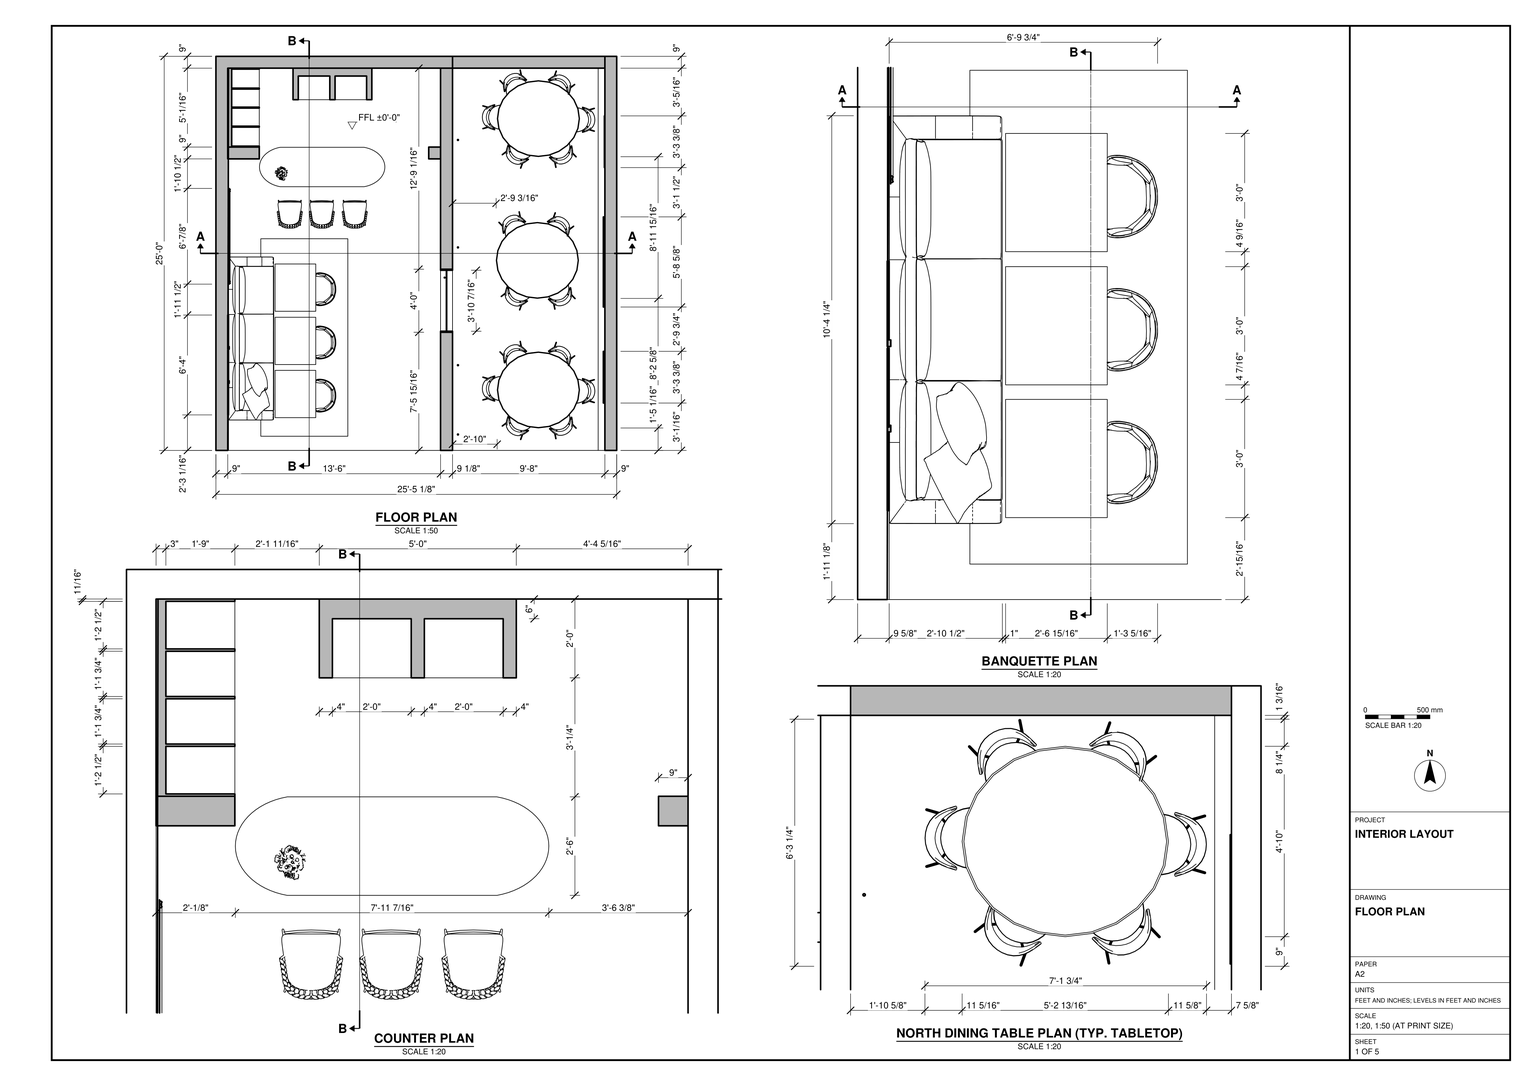
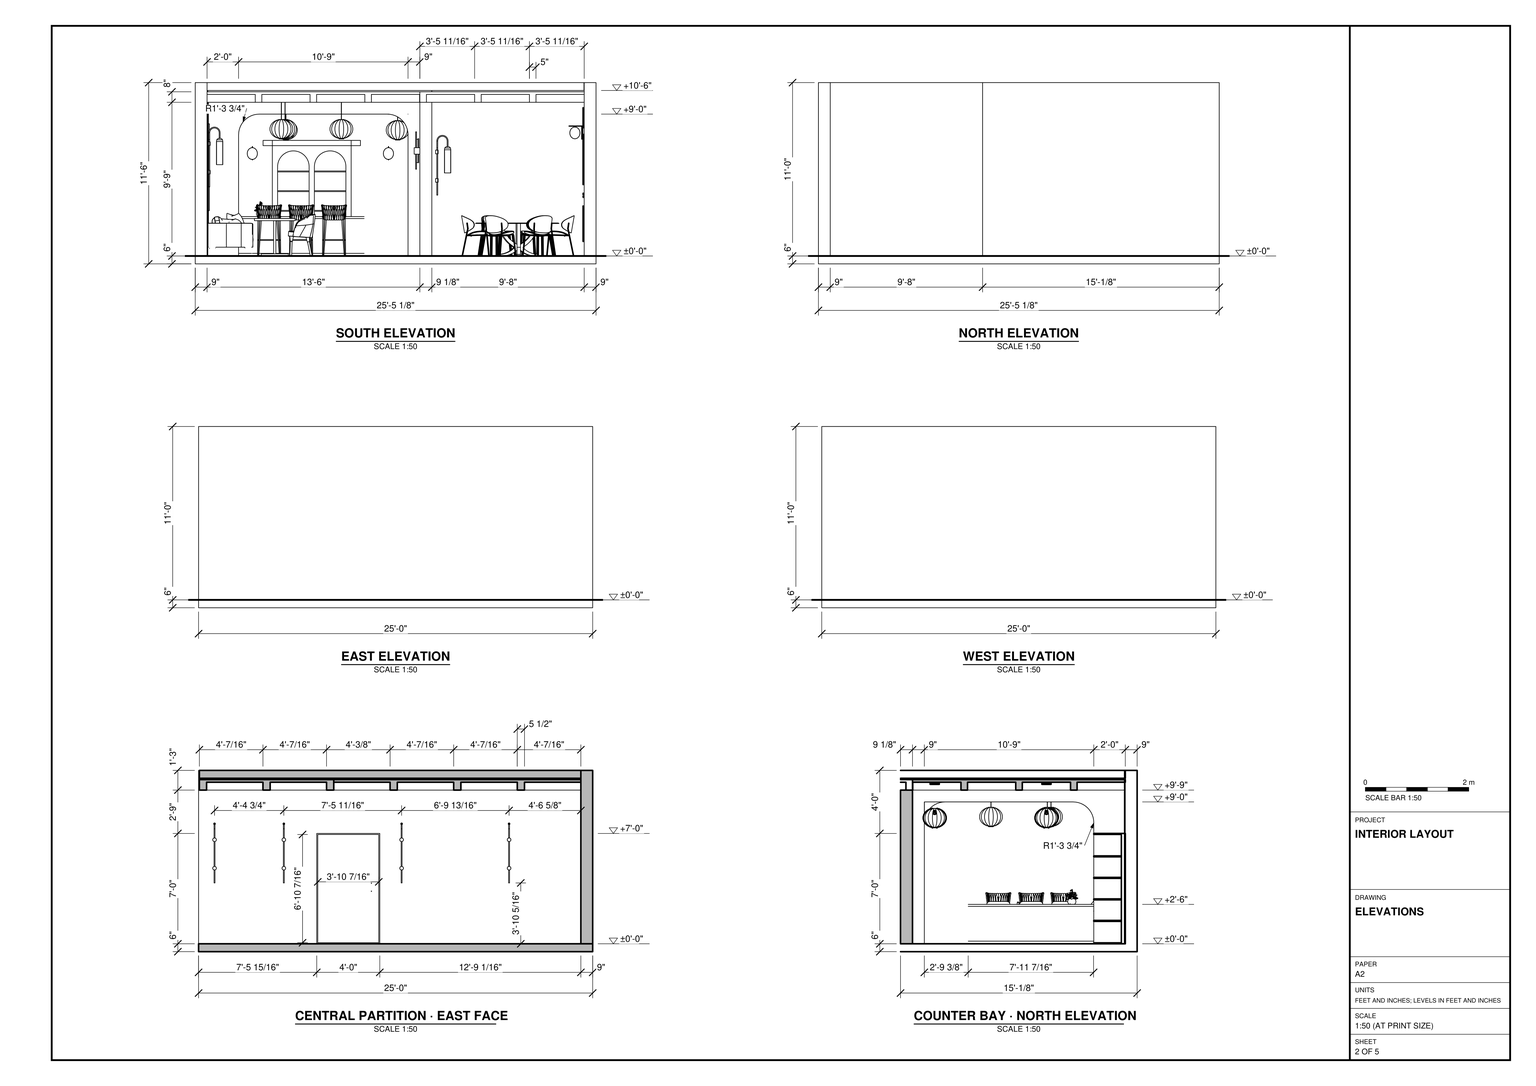
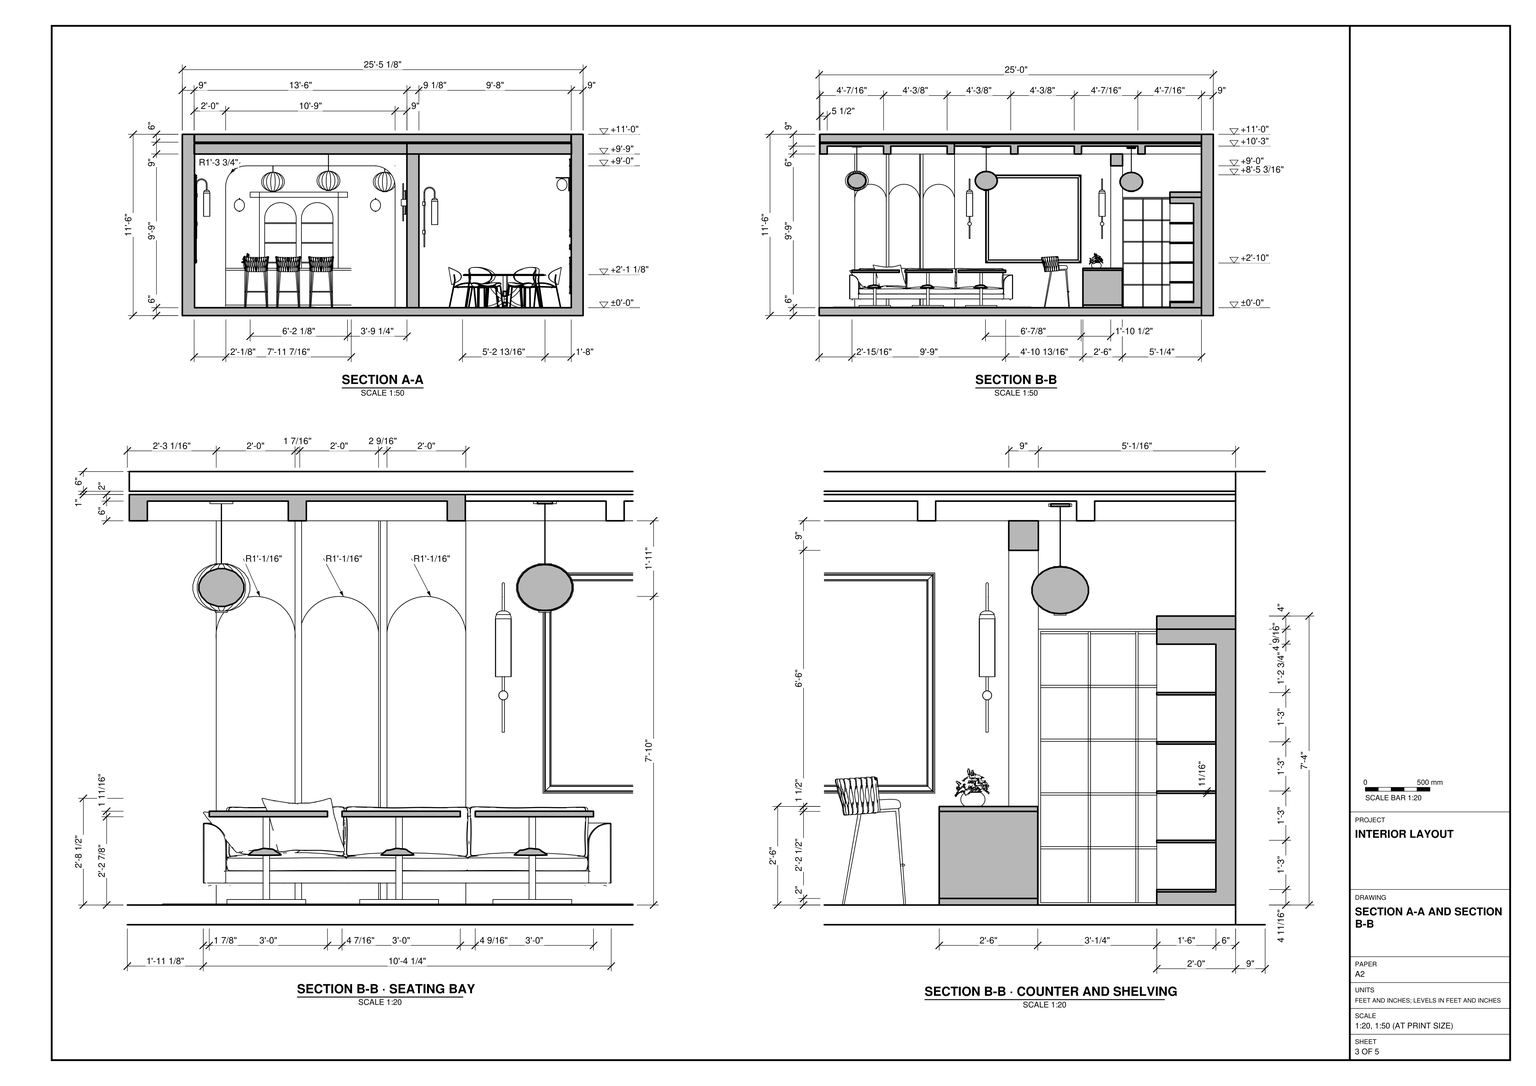
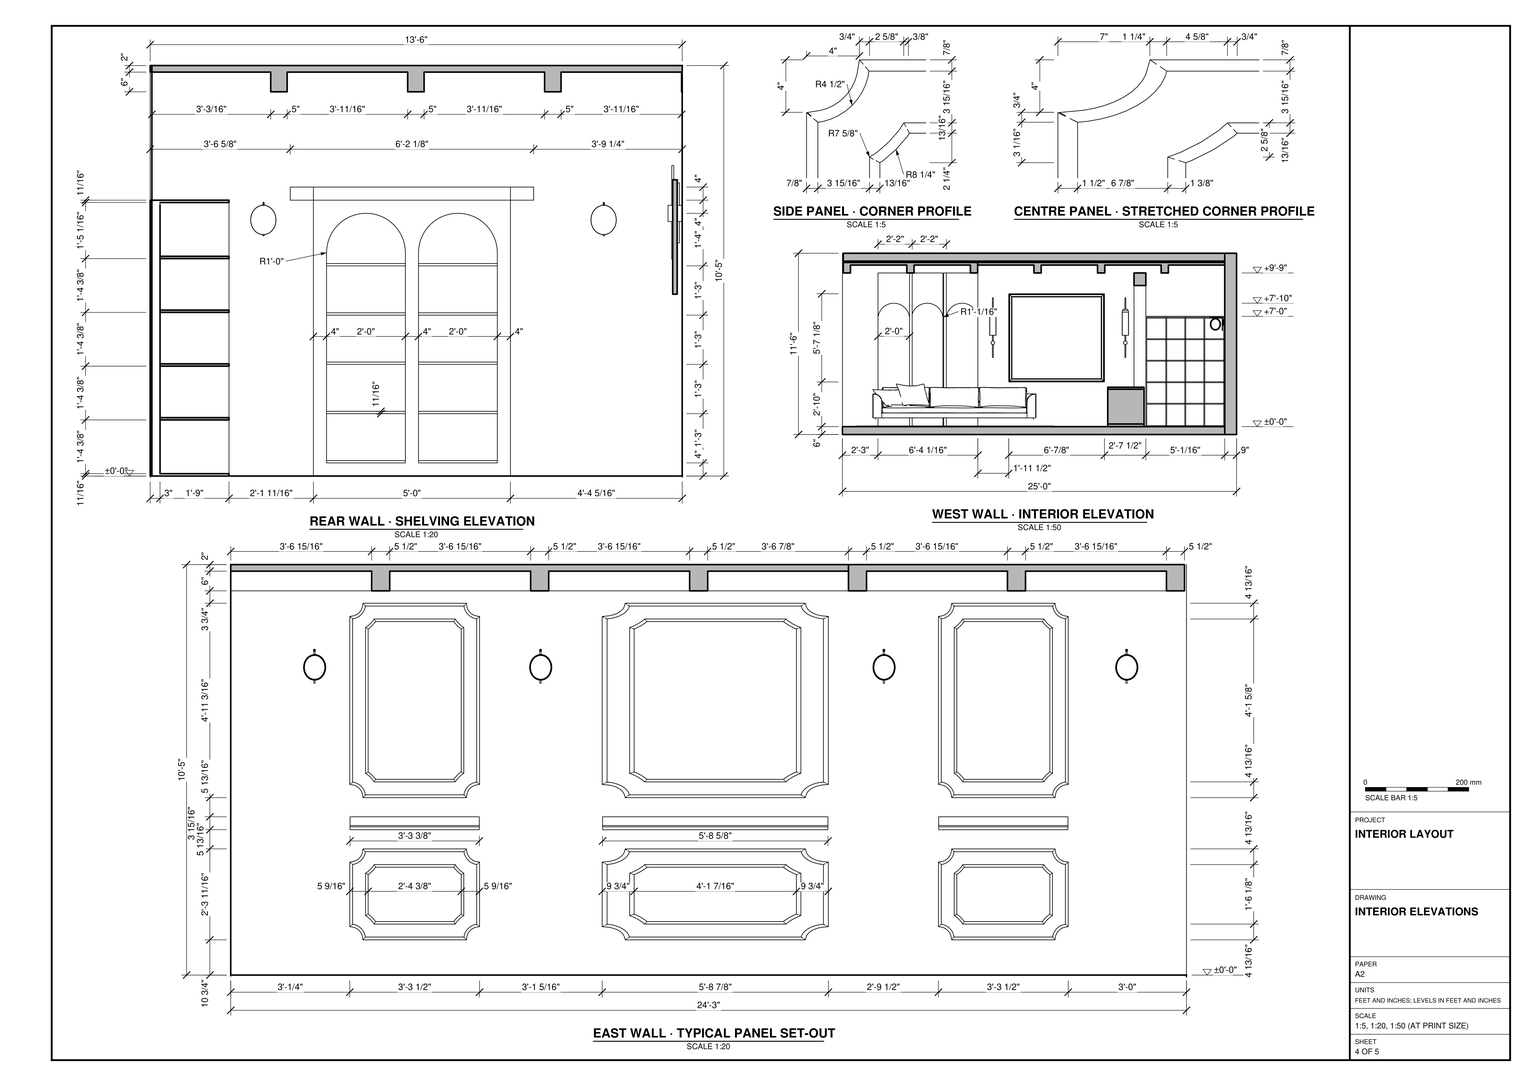
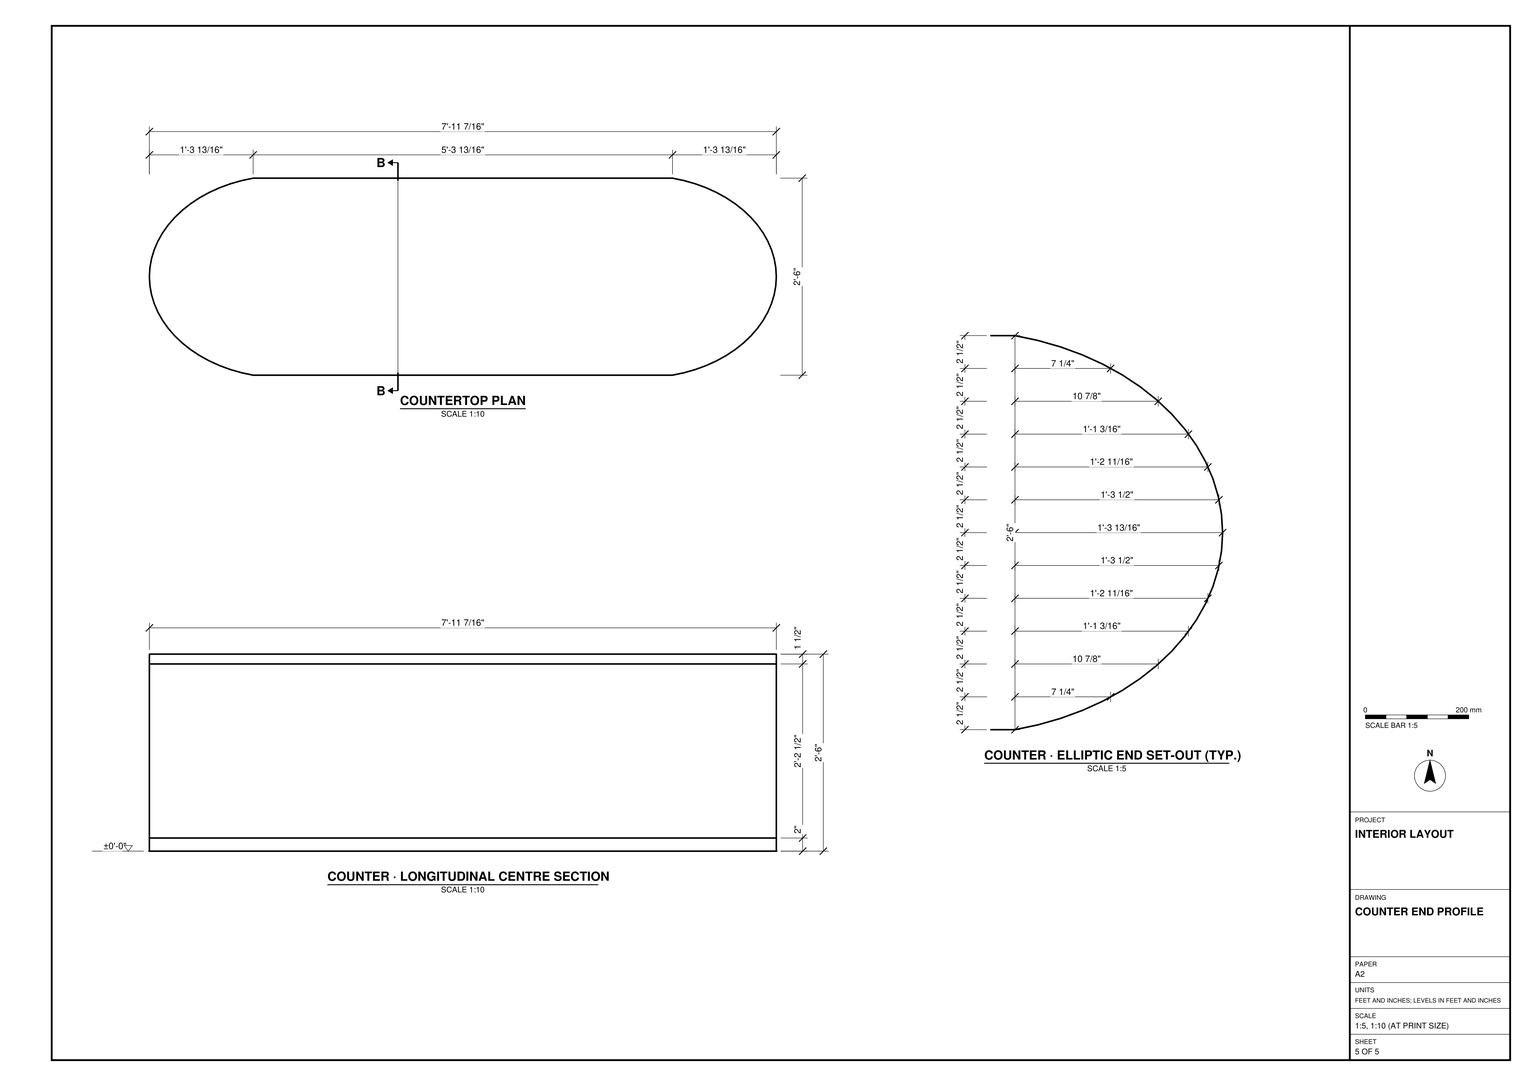
Build the single-storey dining interior in SketchUp from task_files/diagram_01.pdf. Work in feet and inches. The model is 25'-5 1/8" wide from west to east, 25'-0" deep from south to north and 11'-6" high overall. Set the finished floor at ±0'-0".

Model the floor slab, the 9" north, east and west walls, and the roof slab with its ceiling framing. Leave the south side open as drawn. Run the 9 1/8" central partition north to south, with a passage between the wider west bay and the narrower east bay.

At the north end of the west bay, model the rounded-end counter with stools on its south side. Include the shelving beside the counter and the paired arch-headed shelves behind it. Farther south along the west wall, place the banquette against the arched wall panels, with rectangular pedestal tables and chairs facing the bench. Arrange the round dining tables in a north–south row in the east bay, following the chair layouts on the floor plan. For decor and loose items such as lights, cushions and the countertop arrangement, any suitable library components may be used.

Keep shell elements and individual pieces of furniture and joinery in separate groups or components, and use components for repeated parts. Save one SketchUp model as output_files/dining_interior_with_a_counter_and_banquette_seating.skp.

# SketchUp Ruby script. Lengths in inches.
U = 1.inch
M = Sketchup.active_model
def pt(a) = Geom::Point3d.new(a.map { |v| v * U })
def face(e, loops, mat)
  f = e.add_face(loops[0].map { |a| pt(a) })
  loops[1..].each { |l| e.add_face(l.map { |a| pt(a) }).erase! }
  f.material = f.back_material = mat if mat
  f
end
# faces: each face lists its corners as indices into pts; further lists are holes
def faces(e, pts, list, mat = nil) = list.each { |f| face(e, (f[0].is_a?(Array) ? f : [f]).map { |l| l.map { |i| pts[i] } }, mat) }
# xy, xz, yz: faces in a plane at the given z, y or x. An outline is a flat list of corners, or four numbers for a rectangle; further outlines are holes
def ring(l) = l.size == 4 ? [[l[0], l[1]], [l[2], l[1]], [l[2], l[3]], [l[0], l[3]]] : l.each_slice(2).to_a
def flat(e, list, mat, &to3) = list.each { |f| face(e, (f[0].is_a?(Array) ? f : [f]).map { |l| ring(l).map { |u, v| to3.(u, v) } }, mat) }
def xy(e, z, list, mat = nil) = flat(e, list, mat) { |x, y| [x, y, z] }
def xz(e, y, list, mat = nil) = flat(e, list, mat) { |x, z| [x, y, z] }
def yz(e, x, list, mat = nil) = flat(e, list, mat) { |y, z| [x, y, z] }
def lines(e, pts, list) = list.each { |a, b| e.add_line(pt(pts[a]), pt(pts[b])) }
# prism: a flat outline (further loops are holes) pulled along v
def prism(e, loops, v, mat = nil)
  f = face(e, loops, mat); d = Geom::Vector3d.new(v.map { |x| x * U })
  f.pushpull(f.normal.samedirection?(d) ? d.length : -d.length)
end
def box(e, o, s, mat = nil) = prism(e, [[o, [o[0] + s[0], o[1], o[2]], [o[0] + s[0], o[1] + s[1], o[2]], [o[0], o[1] + s[1], o[2]]]], [0, 0, s[2]], mat)
def at(x, y, z, deg = 0) = Geom::Transformation.translation(pt([x, y, z])) * Geom::Transformation.rotation(ORIGIN, Z_AXIS, deg.degrees)
def axes(o, x, y, z) = Geom::Transformation.new([*x, 0, *y, 0, *z, 0, *pt(o).to_a, 1])
def part(name) = M.definitions.add(name)
# library, detail: a bought-in or finely detailed component or shape, given as its bounding box
def library(name, o, s) = part(name).tap { |d| box(d.entities, o, s) }
def detail(e, o, s) = box(e.add_group.entities, o, s)
def put(e, d, t, mat = nil) = e.add_instance(d, t).tap { |i| i.material = mat if mat }
def group(e, t, mat = nil) = e.add_group.tap { |g| g.transformation = t; g.material = mat if mat }.entities
root = M.entities
M.materials.add("Kit Kat Speckle, Stack (A069AF)").color = [227, 224, 217]
M.materials.add("Medina Ceramic Tile, Stack (9IOSLT)").color = [195, 198, 178]
M.materials.add("White Marble (2TZ0C7)").color = [249, 249, 249]
M.materials.add("[0136_Charcoal]").color = [35, 35, 35]
M.materials.add("[Color A01]").color = [210, 181, 140]
M.materials.add("[Color A01]1").color = [255, 204, 204]
M.materials.add("[Color A02]").color = [255, 153, 153]
M.materials.add("[Translucent Glass Gray]").color = [128, 128, 128]
M.materials["[Translucent Glass Gray]"].alpha = 0.5
M.materials.add("[Wood Cherry Original]").color = [150, 85, 41]
M.materials.add("download (11)").color = [125, 112, 90]
c1 = library("stool",[-9.63,-9.64,-0.05],[19.26,21.43,39.06])
c2 = library("WALL+MOLDING+DESIGN (1)",[0,-1.07,0],[102.625,1.07,94.5625])
c3 = library("中式吊燈Nelson_Saucer",[-12.41,-4.96,14.6],[17.37,17.37,33.9])
c4 = library("wall+light+(2)",[66.69,10.19,56.48],[12.57,11.01,12.92])
c5 = library("Wall+light (1)",[0,-2.43,0],[11.56,4.86,45.53])
c6 = library("marble+wall+light",[1.77,1.13,0],[2.91,3.55,23.375])
c7 = part("Wall+painting+6")
g1 = group(c7.entities,at(963.18,181.64,0))
xy(g1,0.39,[[0.39,0,12.2,0.79]],"[0136_Charcoal]")
xy(g1,0.98,[[0.98,0,11.61,0.39]],"[0136_Charcoal]")
xy(g1,19.84,[[0.98,0,11.61,0.39]],"[0136_Charcoal]")
xy(g1,20.43,[[0.39,0,12.2,0.79]],"[0136_Charcoal]")
xz(g1,0,[[[0.39,0.39,12.2,20.43],[0.98,0.98,11.61,19.84]]],"[0136_Charcoal]")
xz(g1,0.39,[[0.98,0.98,11.61,19.84]],"download (11)")
xz(g1,0.79,[[0.39,0.39,12.2,20.43]])
yz(g1,0.39,[[0,0.39,0.79,20.43]],"[0136_Charcoal]")
yz(g1,0.98,[[0,0.98,0.39,19.84]],"[0136_Charcoal]")
yz(g1,11.61,[[0,0.98,0.39,19.84]],"[0136_Charcoal]")
yz(g1,12.2,[[0,0.39,0.79,20.43]],"[0136_Charcoal]")
c8 = library("Vase_Flowers_22.skp",[-5.3,-7.7,-1.52],[10.79,13.24,11.97])
c9 = library("Group\#52",[0,0,0],[0.41,39.51,102.51])
c10 = library("Group\#44",[0,0,0],[0.41,39.51,102.51])
c11 = library("Group\#7",[0,0,0],[72,30,30])
c12 = library("Group\#10",[-7.0625,0,0],[74.125,24,88])
c13 = part("Group\#13")
prism(c13.entities,[[[0,0,0.71],[0,58.65,0.71],[0,58.65,0],[0,44.16,0],[0,43.45,0],[0,29.68,0],[0,28.97,0],[0,15.19,0],[0,14.48,0],[0,0,0]]],[21,0,0])
c14 = library("Group\#23",[0,-2.33,0],[81.74,126.56,34.23])
c15 = library("3-POIGNEE CLC2",[-4.82,-0.26,0],[9.64,0.52,1.61])
c16 = library("Group\#32",[-2.34,-3.4,0],[85.74,76.61,30.73])
c17 = library("Group\#33",[-2.34,-3.4,0],[85.74,76.61,30.73])
c18 = library("Group\#31",[8.99,-3.4,0],[62.82,76.61,30.73])
c19 = part("Group\#14")
xy(c19.entities,0,[[0,0,0.1,24]])
xz(c19.entities,0,[[0,0,0.1,83.01]])
xz(c19.entities,24,[[0,0,0.1,83.01]])
yz(c19.entities,0,[[0,0,0,83.01,0.02,83.35,0.26,84.67,0.64,85.96,1.16,87.2,1.82,88.38,2.6,89.47,3.5,90.47,4.51,91.36,5.61,92.14,6.79,92.79,8.03,93.3,9.33,93.67,10.66,93.9,12,93.97,13.34,93.9,14.67,93.67,15.97,93.3,17.21,92.79,18.39,92.14,19.49,91.36,20.5,90.47,21.4,89.47,22.18,88.38,22.84,87.2,23.36,85.96,23.74,84.67,23.98,83.35,24,83.01,24,0]])
yz(c19.entities,0.1,[[0,0,24,0,24,83.01,23.98,83.35,23.74,84.67,23.36,85.96,22.84,87.2,22.18,88.38,21.4,89.47,20.5,90.47,19.49,91.36,18.39,92.14,17.21,92.79,15.97,93.3,14.67,93.67,13.34,93.9,12,93.97,10.66,93.9,9.33,93.67,8.03,93.3,6.79,92.79,5.61,92.14,4.51,91.36,3.5,90.47,2.6,89.47,1.82,88.38,1.16,87.2,0.64,85.96,0.26,84.67,0.02,83.35,0,83.01]],"[Color A02]")
p = [[0,0.02,83.35],[0,0,83.01],[0.1,0,83.01],[0.1,0.02,83.35],[0,24,83.01],[0,23.98,83.35],
  [0.1,23.98,83.35],[0.1,24,83.01],[0,0.26,84.67],[0.1,0.26,84.67],[0,23.74,84.67],[0.1,23.74,84.67],
  [0,0.64,85.96],[0.1,0.64,85.96],[0,23.36,85.96],[0.1,23.36,85.96],[0,1.16,87.2],[0.1,1.16,87.2],
  [0,22.84,87.2],[0.1,22.84,87.2],[0,1.82,88.38],[0.1,1.82,88.38],[0,22.18,88.38],[0.1,22.18,88.38],
  [0,2.6,89.47],[0.1,2.6,89.47],[0,21.4,89.47],[0.1,21.4,89.47],[0,3.5,90.47],[0.1,3.5,90.47],
  [0,20.5,90.47],[0.1,20.5,90.47],[0,4.51,91.36],[0.1,4.51,91.36],[0,19.49,91.36],[0.1,19.49,91.36],
  [0,5.61,92.14],[0.1,5.61,92.14],[0,18.39,92.14],[0.1,18.39,92.14],[0,6.79,92.79],[0.1,6.79,92.79],
  [0,17.21,92.79],[0.1,17.21,92.79],[0,8.03,93.3],[0.1,8.03,93.3],[0,15.97,93.3],[0.1,15.97,93.3],
  [0,9.33,93.67],[0.1,9.33,93.67],[0,14.67,93.67],[0.1,14.67,93.67],[0,10.66,93.9],[0.1,10.66,93.9],
  [0,13.34,93.9],[0.1,13.34,93.9],[0,12,93.97],[0.1,12,93.97]]
faces(c19.entities,p,[[0,1,2,3],[4,5,6,7],[8,0,3,9],[5,10,11,6],[12,8,9,13],[10,14,15,11],[16,12,13,17],[14,18,19,15],
  [20,16,17,21],[18,22,23,19],[24,20,21,25],[22,26,27,23],[28,24,25,29],[26,30,31,27],[32,28,29,33],[30,34,35,31],
  [36,32,33,37],[34,38,39,35],[40,36,37,41],[38,42,43,39],[44,40,41,45],[42,46,47,43],[48,44,45,49],[46,50,51,47],
  [52,48,49,53],[50,54,55,51],[56,52,53,57],[54,56,57,55]])
c20 = part("Group\#1")
prism(c20.entities,[[[0,7.46,117],[0,12,117],[0,24,117],[0,24,0],[0,0,0],[0,0,117]]],[0.5,0,0])
put(c20.entities,c19,at(0.5,0,0))
put(root,c1,at(56.22,180.9,6.05,180))
put(root,c1,at(80.59,180.9,6.05,180))
put(root,c1,at(105.66,180.9,6.05,180))
put(root,c2,axes([10.05,126.58,40.03],[0,0.71,0],[-0.71,0,0],[0,0,0.71]))
put(root,c3,at(69.29,24.93,80.5))
put(root,c3,at(114.97,75.55,80.5))
put(root,c3,at(72.1,123.44,80.5))
put(root,c4,axes([362.8,76.39,26.6875],[-1,0,0],[0,1,0],[0,0,1.16]))
put(root,c4,axes([362.8,2.49,26.6875],[-1,0,0],[0,1,0],[0,0,1.16]))
put(root,c4,axes([362.8,180.95,26.6875],[-1,0,0],[0,1,0],[0,0,1.16]))
put(root,c4,axes([362.8,249.79,26.6875],[-1,0,0],[0,1,0],[0,0,1.16]))
put(root,c4,axes([131.375,357.72,10.97],[0,-1,0],[1,0,0],[0,0,1.16]))
put(root,c5,at(9.44,215.36,58.625))
put(root,c5,at(9.44,114.49,58.625))
put(root,c3,at(114.97,171.74,80.5))
put(root,c4,axes([27.76,357.72,10.97],[0,-1,0],[1,0,0],[0,0,1.16]))
put(root,c3,at(72.74,233.9,79.66))
put(root,c3,at(157.82,233.9,79.66))
put(root,c6,axes([165.29,286.79,72.05],[0,-1.22,0],[1.22,0,0],[0,0,1.22]))
put(root,c7,axes([-147.72,2437.36,60.6875],[0,-2.24296,0],[1.73873,0,0],[0,0,1.73873]))
put(root,c6,axes([165.29,247.23,72.05],[0,-1.22,0],[1.22,0,0],[0,0,1.22]))
put(root,c5,at(182.99,64.9,52.33))
put(root,c5,at(182.99,154.5625,52.33))
put(root,c5,at(182.99,236.375,52.33))
put(root,c5,at(182.99,12.15,52.33))
put(root,c6,axes([165.29,202.35,72.05],[0,-1.22,0],[1.22,0,0],[0,0,1.22]))
put(root,c6,axes([165.29,157.79,72.05],[0,-1.22,0],[1.22,0,0],[0,0,1.22]))
put(root,c6,axes([165.29,77.24,72.05],[0,-1.22,0],[1.22,0,0],[0,0,1.22]))
put(root,c6,axes([165.29,19.74,72.05],[0,-1.22,0],[1.22,0,0],[0,0,1.22]))
put(root,c8,axes([49.73,211.03,36],[1.17,0,0],[0,1.35896,0],[0,0,1.17]))
g2 = group(root,at(0,120.02,6),"[Color A01]1")
xy(g2,-6,[[0,-120.02,9,-120.02,9,171,171,171,171,-120.02,291,-120.02,291,180,0,180],[9,-120.02,171,171],[291,-120.02,296.11,180],[296.11,-120.02,305.11,180]])
xy(g2,0,[[9,-120.02,9.6,-120.02,9.6,171],[291,-120.02,296.11,171],[180.125,171,291,180],[291,171,296.11,180]])
xy(g2,0,[[9.6,-120.02,291,171]],"White Marble (2TZ0C7)")
xy(g2,132,[[0,-120.02,9,-120.02,9,171,180.125,171,180.125,180,0,180],[9,-120.02,9.6,171,9,171],[296.11,-120.02,305.11,180],[180.125,171,296.11,180]])
xz(g2,-120.02,[[0,-6,305.11,-6,305.11,132,296.11,132,296.11,0,9,0,9,132,0,132]])
xz(g2,171,[[9,-6,171,-6,171,0,9.6,0,9.6,132,9,132],[9.6,0,180.125,132],[180.125,123,296.11,132]])
xz(g2,171,[[180.125,0,296.11,123]],"Kit Kat Speckle, Stack (A069AF)")
xz(g2,180,[[0,-6,0,132,180.125,132,180.125,0,296.11,0,296.11,132,305.11,132,305.11,-6],[180.125,0,296.11,132]])
yz(g2,0,[[-120.02,-6,180,132]])
yz(g2,180.125,[[171,0,180,132]])
yz(g2,296.11,[[-120.02,0,171,132],[171,0,180,132]])
yz(g2,305.11,[[-120.02,-6,180,132]])
p = [[9,-120.02,0],[9.6,171,0],[9.6,171,132],[9,-120.02,132],[296.11,171,0],[296.11,171,-6]]
faces(g2,p,[[0,1,2,3]])
lines(g2,p,[[4,5]])
put(g2,c9,at(295.7,95.24,10.73))
put(g2,c10,at(294.91,-84.01,10.73))
put(g2,c9,axes([294.91,-10.98,10.73],[1,0,0],[0,1.743,0],[0,0,1]))
g3 = group(root,at(9,120.02,138))
box(g3,[0,-119.42,-6],[286.92,290.42,6])
put(root,c11,axes([33.15,200.78,6],[1.32572,0,0],[0,1,0],[0,0,1]),"[Color A02]")
put(root,c12,at(58.7,267.02,6))
g4 = group(root,at(9,230.96,6),"[Wood Cherry Original]")
xy(g4,0,[[0,0,24,60.0625]])
xy(g4,0.71,[[3,0.71,24,15.19],[3,15.9,24,29.68],[3,30.39,24,44.16],[3,44.87,24,59.35]])
xy(g4,83.29,[[3,0.71,3.71,15.19],[3.71,0.71,24,15.19],[3,15.19,3.71,15.9],[3.71,15.19,24,15.9],[3,15.9,3.71,29.68],
  [3.71,15.9,24,29.68],[3,29.68,3.71,30.39],[3.71,29.68,24,30.39],[3,30.39,3.71,44.16],[3.71,30.39,24,44.16],
  [3,44.16,3.71,44.87],[3.71,44.16,24,44.87],[3,44.87,3.71,59.35],[3.71,44.87,24,59.35]])
xy(g4,84,[[0,0,24,60.0625]])
xz(g4,0,[[0,0,24,84]])
xz(g4,0.71,[[3,0.71,24,83.29]])
xz(g4,15.19,[[3,0.71,24,83.29]])
xz(g4,15.9,[[3,0.71,24,83.29]])
xz(g4,29.68,[[3,0.71,24,83.29]])
xz(g4,30.39,[[3,0.71,24,83.29]])
xz(g4,44.16,[[3,0.71,24,83.29]])
xz(g4,44.87,[[3,0.71,24,83.29]])
xz(g4,59.35,[[3,0.71,24,83.29]])
xz(g4,60.0625,[[0,0,24,84]])
yz(g4,0,[[0,0,60.0625,84]])
yz(g4,3,[[0.71,0.71,15.19,82.58],[15.9,0.71,29.68,82.58],[30.39,0.71,44.16,82.58],[44.87,0.71,59.35,82.58],[15.19,82.58,15.9,83.29],
  [29.68,82.58,30.39,83.29],[44.16,82.58,44.87,83.29]])
yz(g4,24,[[[0,0,60.0625,84],[0.71,0.71,59.35,83.29]],[15.19,0.71,15.9,83.29],[29.68,0.71,30.39,83.29],[44.16,0.71,44.87,83.29]])
put(g4,c13,at(3,0.71,66.21))
put(g4,c13,at(3,0.71,49.83))
put(g4,c13,at(3,0.71,33.46))
put(g4,c13,at(3,0.71,17.08))
g5 = group(root,at(9,221.96,0))
xy(g5,6,[[0,0,24,9],[153,0,162,9]])
xy(g5,114,[[39.74,0,137.26,9],[137.26,0,152.93,9],[152.93,0,153,9]])
xy(g5,123,[[0,0,162,9]])
xz(g5,0,[[0,6,24,6,24,98.26,24.13,100.3125,24.54,102.33,25.2,104.28,26.11,106.13,27.25,107.84,28.61,109.39,30.16,110.75,31.87,111.89,33.72,112.8,35.67,113.46,37.6875,113.87,39.74,114,153,114,153,6,162,6,162,123,0,123],[152.93,99.29,152.93,114,137.26,114,139.3125,113.87,141.33,113.46,143.28,112.8,145.13,111.89,146.84,110.75,148.39,109.39,149.75,107.84,150.89,106.13,151.8,104.28,152.46,102.33,152.87,100.3125]])
xz(g5,9,[[0,6,0,123,162,123,162,6,153,6,153,114,39.74,114,37.6875,113.87,35.67,113.46,33.72,112.8,31.87,111.89,30.16,110.75,28.61,109.39,27.25,107.84,26.11,106.13,25.2,104.28,24.54,102.33,24.13,100.3125,24,98.26,24,6],[153,98.26,152.93,99.29,152.93,114,153,114],[152.93,99.29,152.87,100.3125,152.46,102.33,151.8,104.28,150.89,106.13,149.75,107.84,148.39,109.39,146.84,110.75,145.13,111.89,143.28,112.8,141.33,113.46,139.3125,113.87,137.26,114,152.93,114]])
yz(g5,0,[[0,6,9,123]])
yz(g5,24,[[0,6,9,98.26]])
yz(g5,152.93,[[0,99.29,9,114]])
yz(g5,153,[[0,6,9,114]])
yz(g5,162,[[0,6,9,123]])
p = [[24.13,0,100.3125],[24,0,98.26],[24,9,98.26],[24.13,9,100.3125],[152.87,9,100.3125],[152.93,9,99.29],
  [152.93,0,99.29],[152.87,0,100.3125],[24.54,0,102.33],[24.54,9,102.33],[152.46,9,102.33],[152.46,0,102.33],
  [25.2,0,104.28],[25.2,9,104.28],[151.8,9,104.28],[151.8,0,104.28],[26.11,0,106.13],[26.11,9,106.13],
  [150.89,9,106.13],[150.89,0,106.13],[27.25,0,107.84],[27.25,9,107.84],[149.75,9,107.84],[149.75,0,107.84],
  [28.61,0,109.39],[28.61,9,109.39],[148.39,9,109.39],[148.39,0,109.39],[30.16,0,110.75],[30.16,9,110.75],
  [146.84,9,110.75],[146.84,0,110.75],[31.87,0,111.89],[31.87,9,111.89],[145.13,9,111.89],[145.13,0,111.89],
  [33.72,0,112.8],[33.72,9,112.8],[143.28,9,112.8],[143.28,0,112.8],[35.67,0,113.46],[35.67,9,113.46],
  [141.33,9,113.46],[141.33,0,113.46],[37.6875,0,113.87],[37.6875,9,113.87],[139.3125,9,113.87],[139.3125,0,113.87],
  [39.74,0,114],[39.74,9,114],[137.26,9,114],[137.26,0,114]]
faces(g5,p,[[0,1,2,3],[4,5,6,7],[8,0,3,9],[10,4,7,11],[12,8,9,13],[14,10,11,15],[16,12,13,17],[18,14,15,19],
  [20,16,17,21],[22,18,19,23],[24,20,21,25],[26,22,23,27],[28,24,25,29],[30,26,27,31],[32,28,29,33],[34,30,31,35],
  [36,32,33,37],[38,34,35,39],[40,36,37,41],[42,38,39,43],[44,40,41,45],[46,42,43,47],[48,44,45,49],[50,46,47,51]])
put(root,c14,at(9.6,23.11,6),"[Wood Cherry Original]")
g6 = group(root,at(171,0,6))
xy(g6,0,[[0,0,9.125,89.96],[0,137.96,9.125,291.02]])
xy(g6,117,[[0,0,9.125,291.02]])
xz(g6,0,[[0,0,9.125,117]])
xz(g6,89.96,[[0,0,9.125,84]])
xz(g6,137.96,[[0,0,9.125,84]])
xz(g6,291.02,[[0,0,9.125,117]])
yz(g6,0,[[0,0,0,117,291.02,117,291.02,0,137.96,0,137.96,84,89.96,84,89.96,0]],"[Color A01]")
yz(g6,9.125,[[0,0,89.96,0,89.96,84,137.96,84,137.96,0,291.02,0,291.02,117,0,117]])
put(g6,c15,axes([4.44,131.58,43.07],[0,0,1],[0,1,0],[-1,0,0]))
g7 = group(g6,at(0,89.96,84))
xy(g7,-84,[[0,0,9.125,48]])
xy(g7,-83.21,[[0,0.79,4.5625,47.21],[4.5625,0.79,9.125,47.21]])
xy(g7,-0.79,[[0,0.79,4.5625,47.21],[4.5625,0.79,9.125,47.21]])
xy(g7,0,[[0,0,9.125,48]])
xz(g7,0,[[0,-84,9.125,0]])
xz(g7,0.79,[[0,-83.21,4.5625,-0.79],[4.5625,-83.21,9.125,-0.79]])
xz(g7,47.21,[[0,-83.21,4.5625,-0.79],[4.5625,-83.21,9.125,-0.79]])
xz(g7,48,[[0,-84,9.125,0]])
yz(g7,0,[[[0,-84,48,0],[0.79,-83.21,47.21,-0.79]]])
yz(g7,9.125,[[[0,-84,48,0],[0.79,-83.21,47.21,-0.79]]])
g8 = group(g7,at(4.5625,0.79,-83.21),"[Translucent Glass Gray]")
box(g8,[-0.12,0,0],[0.24,46.43,82.43])
g9 = group(root,at(34.17,10.8,6),"Medina Ceramic Tile, Stack (9IOSLT)")
xy(g9,0,[[0,0,66.25,150.375]])
xy(g9,0.2,[[0,0,66.25,150.375]],"Medina Ceramic Tile, Stack (9IOSLT)")
xz(g9,0,[[0,0,66.25,0.2]])
xz(g9,150.375,[[0,0,66.25,0.2]])
yz(g9,0,[[0,0,150.375,0.2]])
yz(g9,66.25,[[0,0,150.375,0.2]])
put(root,c16,at(205.1,217.28,6))
put(root,c17,at(205.1,10.71,6))
put(root,c18,at(204.32,109.36,6))
g10 = group(root,at(9,0.6,123))
g11 = group(g10,at(125.3,0,0))
g12 = group(g11,at(0,102.32,8))
xy(g12,-8,[[[36.7,0,41.7,0,41.7,42.86,78.41,42.86,78.41,0,83.41,0,83.41,42.86,120.11,42.86,120.11,0,125.11,0,125.11,42.86,161.8125,42.86,161.8125,0,162,0,162,188.1,161.8125,188.1,161.8125,145.1875,125.11,145.1875,125.11,188.1,120.11,188.1,120.11,145.1875,83.41,145.1875,83.41,188.1,78.41,188.1,78.41,145.1875,41.7,145.1875,41.7,188.1,36.7,188.1],[83.41,48.36,120.11,91.28],[125.11,96.78,161.8125,139.6875],[41.7,96.78,78.41,139.6875],[83.41,96.78,120.11,139.6875],[41.7,48.36,78.41,91.28],[125.11,48.36,161.8125,91.28]]])
xy(g12,-2,[[41.7,0,78.41,42.86],[83.41,0,120.11,42.86],[125.11,0,161.8125,42.86],[41.7,48.36,78.41,91.28],[83.41,48.36,120.11,91.28],
  [125.11,48.36,161.8125,91.28],[41.7,96.78,78.41,139.6875],[83.41,96.78,120.11,139.6875],[125.11,96.78,161.8125,139.6875],[41.7,145.1875,78.41,188.1],
  [83.41,145.1875,120.11,188.1],[125.11,145.1875,161.8125,188.1]])
xy(g12,0,[[36.7,0,162,188.1]])
xz(g12,0,[[36.7,-8,36.7,0,162,0,162,-8,161.8125,-8,161.8125,-2,125.11,-2,125.11,-8,120.11,-8,120.11,-2,83.41,-2,83.41,-8,78.41,-8,78.41,-2,41.7,-2,41.7,-8]])
xz(g12,42.86,[[41.7,-8,78.41,-2],[83.41,-8,120.11,-2],[125.11,-8,161.8125,-2]])
xz(g12,48.36,[[41.7,-8,78.41,-2],[83.41,-8,120.11,-2],[125.11,-8,161.8125,-2]])
xz(g12,91.28,[[41.7,-8,78.41,-2],[83.41,-8,120.11,-2],[125.11,-8,161.8125,-2]])
xz(g12,96.78,[[41.7,-8,78.41,-2],[83.41,-8,120.11,-2],[125.11,-8,161.8125,-2]])
xz(g12,139.6875,[[41.7,-8,78.41,-2],[83.41,-8,120.11,-2],[125.11,-8,161.8125,-2]])
xz(g12,145.1875,[[41.7,-8,78.41,-2],[83.41,-8,120.11,-2],[125.11,-8,161.8125,-2]])
xz(g12,188.1,[[36.7,-8,41.7,-8,41.7,-2,78.41,-2,78.41,-8,83.41,-8,83.41,-2,120.11,-2,120.11,-8,125.11,-8,125.11,-2,161.8125,-2,161.8125,-8,162,-8,162,0,36.7,0]])
yz(g12,36.7,[[0,-8,42.86,-2],[42.86,-8,48.36,-8,48.36,-2,91.28,-2,91.28,-8,96.78,-8,96.78,-2,139.6875,-2,139.6875,-8,145.1875,-8,145.1875,-2,188.1,-2,188.1,0,0,0,0,-2,42.86,-2],[48.36,-8,91.28,-2],[96.78,-8,139.6875,-2],[145.1875,-8,188.1,-2]])
yz(g12,41.7,[[0,-8,42.86,-2],[48.36,-8,91.28,-2],[96.78,-8,139.6875,-2],[145.1875,-8,188.1,-2]])
yz(g12,78.41,[[0,-8,42.86,-2],[48.36,-8,91.28,-2],[96.78,-8,139.6875,-2],[145.1875,-8,188.1,-2]])
yz(g12,83.41,[[0,-8,42.86,-2],[48.36,-8,91.28,-2],[96.78,-8,139.6875,-2],[145.1875,-8,188.1,-2]])
yz(g12,120.11,[[0,-8,42.86,-2],[48.36,-8,91.28,-2],[96.78,-8,139.6875,-2],[145.1875,-8,188.1,-2]])
yz(g12,125.11,[[0,-8,42.86,-2],[48.36,-8,91.28,-2],[96.78,-8,139.6875,-2],[145.1875,-8,188.1,-2]])
yz(g12,161.8125,[[0,-8,42.86,-2],[48.36,-8,91.28,-2],[96.78,-8,139.6875,-2],[145.1875,-8,188.1,-2]])
yz(g12,162,[[0,-8,188.1,0]])
g13 = group(g11,at(0,-42.86,8))
xy(g13,-8,[[[36.7,42.86,162,145.1875],[83.41,48.36,120.11,91.28],[125.11,96.78,161.8125,139.6875],[41.7,96.78,78.41,139.6875],[83.41,96.78,120.11,139.6875],[41.7,48.36,78.41,91.28],[125.11,48.36,161.8125,91.28]]])
xy(g13,-2,[[41.7,48.36,78.41,91.28],[83.41,48.36,120.11,91.28],[125.11,48.36,161.8125,91.28],[41.7,96.78,78.41,139.6875],[83.41,96.78,120.11,139.6875],
  [125.11,96.78,161.8125,139.6875]])
xy(g13,0,[[36.7,42.86,162,145.1875]])
xz(g13,42.86,[[36.7,-8,36.7,0,162,0,162,-8,161.8125,-8,161.8125,-2,125.11,-2,125.11,-8,120.11,-8,120.11,-2,83.41,-2,83.41,-8,78.41,-8,78.41,-2,41.7,-2,41.7,-8],[41.7,-8,78.41,-2],[83.41,-8,120.11,-2],[125.11,-8,161.8125,-2]])
xz(g13,48.36,[[41.7,-8,78.41,-2],[83.41,-8,120.11,-2],[125.11,-8,161.8125,-2]])
xz(g13,91.28,[[41.7,-8,78.41,-2],[83.41,-8,120.11,-2],[125.11,-8,161.8125,-2]])
xz(g13,96.78,[[41.7,-8,78.41,-2],[83.41,-8,120.11,-2],[125.11,-8,161.8125,-2]])
xz(g13,139.6875,[[41.7,-8,78.41,-2],[83.41,-8,120.11,-2],[125.11,-8,161.8125,-2]])
xz(g13,145.1875,[[36.7,-8,41.7,-8,41.7,-2,78.41,-2,78.41,-8,83.41,-8,83.41,-2,120.11,-2,120.11,-8,125.11,-8,125.11,-2,161.8125,-2,161.8125,-8,162,-8,162,0,36.7,0],[41.7,-8,78.41,-2],[83.41,-8,120.11,-2],[125.11,-8,161.8125,-2]])
yz(g13,36.7,[[42.86,-8,48.36,-8,48.36,-2,91.28,-2,91.28,-8,96.78,-8,96.78,-2,139.6875,-2,139.6875,-8,145.1875,-8,145.1875,0,42.86,0],[48.36,-8,91.28,-2],[96.78,-8,139.6875,-2]])
yz(g13,41.7,[[48.36,-8,91.28,-2],[96.78,-8,139.6875,-2]])
yz(g13,78.41,[[48.36,-8,91.28,-2],[96.78,-8,139.6875,-2]])
yz(g13,83.41,[[48.36,-8,91.28,-2],[96.78,-8,139.6875,-2]])
yz(g13,120.11,[[48.36,-8,91.28,-2],[96.78,-8,139.6875,-2]])
yz(g13,125.11,[[48.36,-8,91.28,-2],[96.78,-8,139.6875,-2]])
yz(g13,161.8125,[[48.36,-8,91.28,-2],[96.78,-8,139.6875,-2]])
yz(g13,162,[[42.86,-8,145.1875,0]])
g14 = group(g10,at(0,0,0))
g15 = group(g14,at(0,102.32,8))
xy(g15,-8,[[[36.7,0,41.7,0,41.7,42.86,78.41,42.86,78.41,0,83.41,0,83.41,42.86,120.11,42.86,120.11,0,125.11,0,125.11,42.86,161.8125,42.86,161.8125,0,162,0,162,188.1,161.8125,188.1,161.8125,145.1875,125.11,145.1875,125.11,188.1,120.11,188.1,120.11,145.1875,83.41,145.1875,83.41,188.1,78.41,188.1,78.41,145.1875,41.7,145.1875,41.7,188.1,36.7,188.1,36.7,145.1875,0,145.1875,0,139.6875,36.7,139.6875,36.7,96.78,0,96.78,0,91.28,36.7,91.28,36.7,48.36,0,48.36,0,42.86,36.7,42.86],[83.41,48.36,120.11,91.28],[125.11,96.78,161.8125,139.6875],[41.7,96.78,78.41,139.6875],[83.41,96.78,120.11,139.6875],[41.7,48.36,78.41,91.28],[125.11,48.36,161.8125,91.28]]])
xy(g15,-2,[[0,0,36.7,42.86],[41.7,0,78.41,42.86],[83.41,0,120.11,42.86],[125.11,0,161.8125,42.86],[0,48.36,36.7,91.28],
  [41.7,48.36,78.41,91.28],[83.41,48.36,120.11,91.28],[125.11,48.36,161.8125,91.28],[0,96.78,36.7,139.6875],[41.7,96.78,78.41,139.6875],
  [83.41,96.78,120.11,139.6875],[125.11,96.78,161.8125,139.6875],[0,145.1875,36.7,188.1],[41.7,145.1875,78.41,188.1],[83.41,145.1875,120.11,188.1],
  [125.11,145.1875,161.8125,188.1]])
xy(g15,0,[[0,0,162,188.1]])
xz(g15,0,[[36.7,-8,36.7,-2,0,-2,0,0,162,0,162,-8,161.8125,-8,161.8125,-2,125.11,-2,125.11,-8,120.11,-8,120.11,-2,83.41,-2,83.41,-8,78.41,-8,78.41,-2,41.7,-2,41.7,-8]])
xz(g15,42.86,[[0,-8,36.7,-2],[41.7,-8,78.41,-2],[83.41,-8,120.11,-2],[125.11,-8,161.8125,-2]])
xz(g15,48.36,[[0,-8,36.7,-2],[41.7,-8,78.41,-2],[83.41,-8,120.11,-2],[125.11,-8,161.8125,-2]])
xz(g15,91.28,[[0,-8,36.7,-2],[41.7,-8,78.41,-2],[83.41,-8,120.11,-2],[125.11,-8,161.8125,-2]])
xz(g15,96.78,[[0,-8,36.7,-2],[41.7,-8,78.41,-2],[83.41,-8,120.11,-2],[125.11,-8,161.8125,-2]])
xz(g15,139.6875,[[0,-8,36.7,-2],[41.7,-8,78.41,-2],[83.41,-8,120.11,-2],[125.11,-8,161.8125,-2]])
xz(g15,145.1875,[[0,-8,36.7,-2],[41.7,-8,78.41,-2],[83.41,-8,120.11,-2],[125.11,-8,161.8125,-2]])
xz(g15,188.1,[[36.7,-8,41.7,-8,41.7,-2,78.41,-2,78.41,-8,83.41,-8,83.41,-2,120.11,-2,120.11,-8,125.11,-8,125.11,-2,161.8125,-2,161.8125,-8,162,-8,162,0,0,0,0,-2,36.7,-2]])
yz(g15,0,[[42.86,-8,48.36,-8,48.36,-2,91.28,-2,91.28,-8,96.78,-8,96.78,-2,139.6875,-2,139.6875,-8,145.1875,-8,145.1875,-2,188.1,-2,188.1,0,0,0,0,-2,42.86,-2]])
yz(g15,36.7,[[0,-8,42.86,-2],[48.36,-8,91.28,-2],[96.78,-8,139.6875,-2],[145.1875,-8,188.1,-2]])
yz(g15,41.7,[[0,-8,42.86,-2],[48.36,-8,91.28,-2],[96.78,-8,139.6875,-2],[145.1875,-8,188.1,-2]])
yz(g15,78.41,[[0,-8,42.86,-2],[48.36,-8,91.28,-2],[96.78,-8,139.6875,-2],[145.1875,-8,188.1,-2]])
yz(g15,83.41,[[0,-8,42.86,-2],[48.36,-8,91.28,-2],[96.78,-8,139.6875,-2],[145.1875,-8,188.1,-2]])
yz(g15,120.11,[[0,-8,42.86,-2],[48.36,-8,91.28,-2],[96.78,-8,139.6875,-2],[145.1875,-8,188.1,-2]])
yz(g15,125.11,[[0,-8,42.86,-2],[48.36,-8,91.28,-2],[96.78,-8,139.6875,-2],[145.1875,-8,188.1,-2]])
yz(g15,161.8125,[[0,-8,42.86,-2],[48.36,-8,91.28,-2],[96.78,-8,139.6875,-2],[145.1875,-8,188.1,-2]])
yz(g15,162,[[0,-8,188.1,0]])
g16 = group(g14,at(0,-42.86,8))
xy(g16,-8,[[[0,42.86,162,42.86,162,145.1875,0,145.1875,0,139.6875,36.7,139.6875,36.7,96.78,0,96.78,0,91.28,36.7,91.28,36.7,48.36,0,48.36],[83.41,48.36,120.11,91.28],[125.11,96.78,161.8125,139.6875],[41.7,96.78,78.41,139.6875],[83.41,96.78,120.11,139.6875],[41.7,48.36,78.41,91.28],[125.11,48.36,161.8125,91.28]]])
xy(g16,-2,[[0,48.36,36.7,91.28],[41.7,48.36,78.41,91.28],[83.41,48.36,120.11,91.28],[125.11,48.36,161.8125,91.28],[0,96.78,36.7,139.6875],
  [41.7,96.78,78.41,139.6875],[83.41,96.78,120.11,139.6875],[125.11,96.78,161.8125,139.6875]])
xy(g16,0,[[0,42.86,162,145.1875]])
xz(g16,42.86,[[0,-8,36.7,-2],[36.7,-8,36.7,-2,0,-2,0,0,162,0,162,-8,161.8125,-8,161.8125,-2,125.11,-2,125.11,-8,120.11,-8,120.11,-2,83.41,-2,83.41,-8,78.41,-8,78.41,-2,41.7,-2,41.7,-8],[41.7,-8,78.41,-2],[83.41,-8,120.11,-2],[125.11,-8,161.8125,-2]])
xz(g16,48.36,[[0,-8,36.7,-2],[41.7,-8,78.41,-2],[83.41,-8,120.11,-2],[125.11,-8,161.8125,-2]])
xz(g16,91.28,[[0,-8,36.7,-2],[41.7,-8,78.41,-2],[83.41,-8,120.11,-2],[125.11,-8,161.8125,-2]])
xz(g16,96.78,[[0,-8,36.7,-2],[41.7,-8,78.41,-2],[83.41,-8,120.11,-2],[125.11,-8,161.8125,-2]])
xz(g16,139.6875,[[0,-8,36.7,-2],[41.7,-8,78.41,-2],[83.41,-8,120.11,-2],[125.11,-8,161.8125,-2]])
xz(g16,145.1875,[[0,-8,36.7,-2],[36.7,-8,41.7,-8,41.7,-2,78.41,-2,78.41,-8,83.41,-8,83.41,-2,120.11,-2,120.11,-8,125.11,-8,125.11,-2,161.8125,-2,161.8125,-8,162,-8,162,0,0,0,0,-2,36.7,-2],[41.7,-8,78.41,-2],[83.41,-8,120.11,-2],[125.11,-8,161.8125,-2]])
yz(g16,0,[[42.86,-8,48.36,-8,48.36,-2,91.28,-2,91.28,-8,96.78,-8,96.78,-2,139.6875,-2,139.6875,-8,145.1875,-8,145.1875,0,42.86,0]])
yz(g16,36.7,[[48.36,-8,91.28,-2],[96.78,-8,139.6875,-2]])
yz(g16,41.7,[[48.36,-8,91.28,-2],[96.78,-8,139.6875,-2]])
yz(g16,78.41,[[48.36,-8,91.28,-2],[96.78,-8,139.6875,-2]])
yz(g16,83.41,[[48.36,-8,91.28,-2],[96.78,-8,139.6875,-2]])
yz(g16,120.11,[[48.36,-8,91.28,-2],[96.78,-8,139.6875,-2]])
yz(g16,125.11,[[48.36,-8,91.28,-2],[96.78,-8,139.6875,-2]])
yz(g16,161.8125,[[48.36,-8,91.28,-2],[96.78,-8,139.6875,-2]])
yz(g16,162,[[42.86,-8,145.1875,0]])
g17 = group(root,at(9,27,6))
put(g17,c20,at(0,52.0625,0))
g18 = group(g17,at(0,50.0625,0))
box(g18,[0,0,0],[1.1,2,117])
g19 = group(g17,at(0,0.0625,0))
xy(g19,0,[[0,0,0.5,24]])
xy(g19,117,[[0,0,0.5,7.46],[0,7.46,0.5,12],[0,12,0.5,24]])
xz(g19,0,[[0,0,0.5,117]])
xz(g19,24,[[0,0,0.5,117]])
yz(g19,0,[[0,0,24,117]])
yz(g19,0.5,[[0,80.66,-0.0625,82,0,83.01,0.02,83.35,0.26,84.67,0.64,85.96,1.16,87.2,1.82,88.38,2.6,89.47,3.5,90.47,4.51,91.36,5.61,92.14,6.79,92.79,8.03,93.3,9.33,93.67,10.66,93.9,12,93.97,13.34,93.9,14.67,93.67,15.97,93.3,17.21,92.79,18.39,92.14,19.49,91.36,20.5,90.47,21.4,89.47,22.18,88.38,22.84,87.2,23.36,85.96,23.74,84.67,23.98,83.35,24,83.01,24.0625,82,24,80.66,24,117,0,117],[0,80.66,0,83.01,-0.0625,82],[24,80.66,24.0625,82,24,83.01]])
put(g19,c19,at(0.5,0,0))
g20 = group(g17,at(0,24.0625,0))
box(g20,[0,0,0],[1.1,2,117])
put(g17,c20,at(0,25.5,0))
